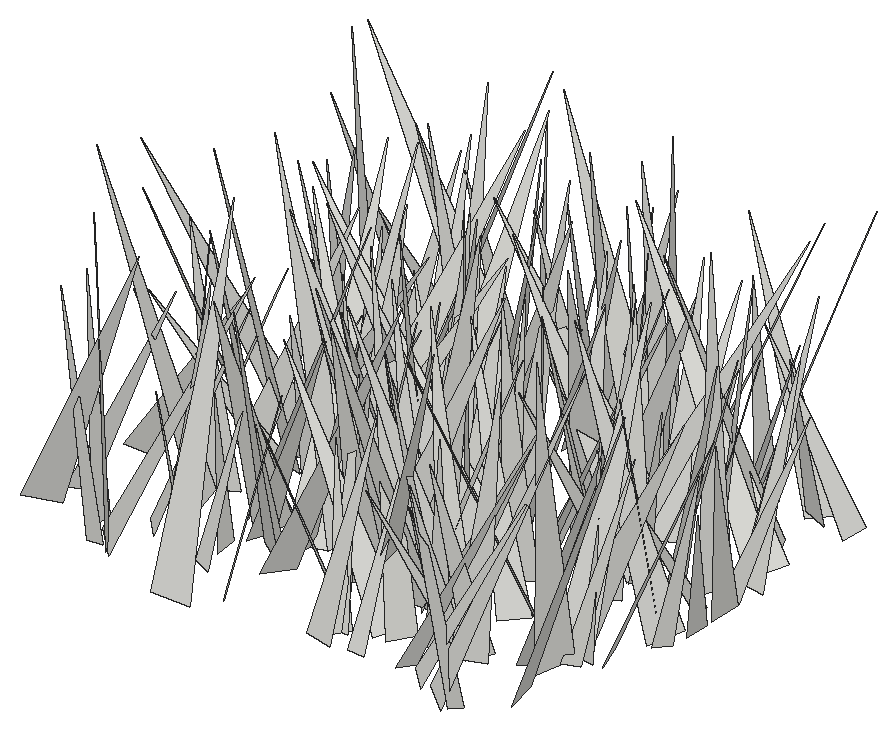
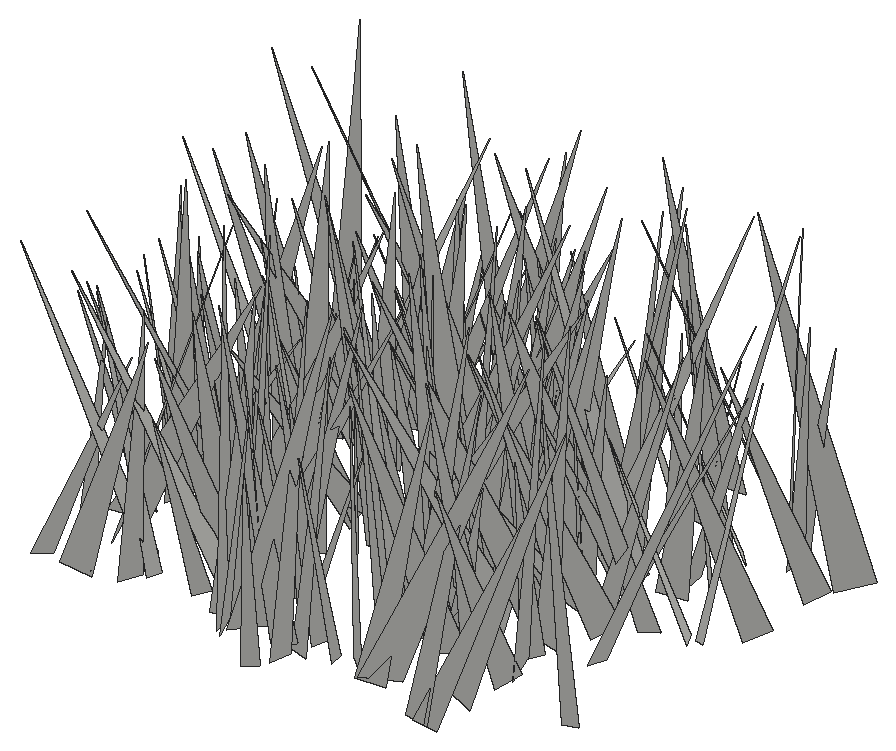
# SketchUp Ruby script. Lengths in inches.
U = 1.inch
M = Sketchup.active_model
def pt(a) = Geom::Point3d.new(a.map { |v| v * U })
def face(e, loops, mat)
  f = e.add_face(loops[0].map { |a| pt(a) })
  loops[1..].each { |l| e.add_face(l.map { |a| pt(a) }).erase! }
  f.material = f.back_material = mat if mat
  f
end
# faces: each face lists its corners as indices into pts; further lists are holes
def faces(e, pts, list, mat = nil) = list.each { |f| face(e, (f[0].is_a?(Array) ? f : [f]).map { |l| l.map { |i| pts[i] } }, mat) }
# xy, xz, yz: faces in a plane at the given z, y or x. An outline is a flat list of corners, or four numbers for a rectangle; further outlines are holes
def ring(l) = l.size == 4 ? [[l[0], l[1]], [l[2], l[1]], [l[2], l[3]], [l[0], l[3]]] : l.each_slice(2).to_a
def flat(e, list, mat, &to3) = list.each { |f| face(e, (f[0].is_a?(Array) ? f : [f]).map { |l| ring(l).map { |u, v| to3.(u, v) } }, mat) }
def xy(e, z, list, mat = nil) = flat(e, list, mat) { |x, y| [x, y, z] }
def xz(e, y, list, mat = nil) = flat(e, list, mat) { |x, z| [x, y, z] }
def yz(e, x, list, mat = nil) = flat(e, list, mat) { |y, z| [x, y, z] }
def lines(e, pts, list) = list.each { |a, b| e.add_line(pt(pts[a]), pt(pts[b])) }
# prism: a flat outline (further loops are holes) pulled along v
def prism(e, loops, v, mat = nil)
  f = face(e, loops, mat); d = Geom::Vector3d.new(v.map { |x| x * U })
  f.pushpull(f.normal.samedirection?(d) ? d.length : -d.length)
end
def box(e, o, s, mat = nil) = prism(e, [[o, [o[0] + s[0], o[1], o[2]], [o[0] + s[0], o[1] + s[1], o[2]], [o[0], o[1] + s[1], o[2]]]], [0, 0, s[2]], mat)
def at(x, y, z, deg = 0) = Geom::Transformation.translation(pt([x, y, z])) * Geom::Transformation.rotation(ORIGIN, Z_AXIS, deg.degrees)
def axes(o, x, y, z) = Geom::Transformation.new([*x, 0, *y, 0, *z, 0, *pt(o).to_a, 1])
def part(name) = M.definitions.add(name)
# library, detail: a bought-in or finely detailed component or shape, given as its bounding box
def library(name, o, s) = part(name).tap { |d| box(d.entities, o, s) }
def detail(e, o, s) = box(e.add_group.entities, o, s)
def put(e, d, t, mat = nil) = e.add_instance(d, t).tap { |i| i.material = mat if mat }
def group(e, t, mat = nil) = e.add_group.tap { |g| g.transformation = t; g.material = mat if mat }.entities
root = M.entities
c1 = part("fur_instance\#9")
p = [[0.8125,0,1.79],[0.67,-0.02,1.48],[0,-0.11,0],[0,0.11,0]]
faces(c1.entities,p,[[0,1,2,3]])
put(root,c1,axes([148.23,232.82,-27.1],[0.29151,4.89673,1.62599],[5.06271,0.04273,-1.03633],[0.99541,-1.65136,4.79468]))
put(root,c1,axes([153.89,233.59,-27.1],[-3.07283,-1.79032,0.75021],[-1.87261,3.10397,-0.26279],[0.51124,0.60869,3.54662]))
put(root,c1,axes([153.01,232.85,-27.1],[3.55975,3.91646,0.08522],[3.79537,-3.41954,-1.38552],[0.97011,-0.99289,5.10792]))
put(root,c1,axes([141.76,233.23,-27.1],[-3.37291,-1.64413,0.77782],[-1.79286,3.28135,-0.83849],[0.30629,1.10194,3.65741]))
put(root,c1,axes([141.93,231.76,-27.1],[-0.24232,8.0833,1.63068],[8.24361,0.27788,-0.15248],[0.20433,-1.625,8.08549]))
put(root,c1,axes([137.36,233.72,-27.1],[-5.46878,-3.64969,2.6695],[-4.02035,5.84198,-0.2491],[2.0696,1.70441,6.57007]))
put(root,c1,axes([154.51,232.05,-27.1],[4.64022,6.0526,0.40907],[6.0581,-4.59639,-0.71102],[0.31728,-0.75645,7.59342]))
put(root,c1,axes([133.34,234.75,-27.1],[5.01421,-5.55154,0.43768],[-5.45899,-4.78379,1.86233],[1.10028,1.565,7.24525]))
put(root,c1,axes([137.01,233.36,-27.1],[-2.00481,-4.221,2.16779],[-4.72189,1.54205,-1.3643],[-0.46899,2.51807,4.46932]))
put(root,c1,axes([155.55,231.93,-27.1],[-6.80362,-1.51626,0.05987],[-1.39466,6.13985,-2.9915],[-0.59797,2.93174,6.29597]))
put(root,c1,axes([148.56,233.77,-27.1],[-3.29969,1.99263,1.18367],[2.06312,3.46364,-0.07948],[1.05601,-0.54058,3.85386]))
put(root,c1,axes([152.93,235.59,-27.1],[-3.89152,-1.38284,0.09587],[-1.31779,3.77936,1.02238],[0.42995,-0.93252,4.00136]))
put(root,c1,axes([153.84,235.57,-27.1],[3.33283,-3.55166,1.19436],[-3.37517,-3.53973,-1.10774],[-1.62758,0.06765,4.74288]))
put(root,c1,axes([143.4,233.2,-27.1],[3.40494,2.47984,0.75094],[2.39973,-3.48584,0.63038],[-0.97714,0.08048,4.16483]))
put(root,c1,axes([152.64,235.5,-27.1],[-3.58815,0.95471,1.93369],[1.59157,3.70529,1.12394],[1.45517,-1.69849,3.5388]))
put(root,c1,axes([148.56,235.94,-27.1],[7.85727,-0.11013,0.63762],[0.0287,-7.70188,-1.68396],[-0.64642,-1.6806,7.67549]))
put(root,c1,axes([156.96,234.15,-27.1],[7.02887,1.41814,0.69885],[1.44367,-7.05544,-0.2028],[-0.64447,-0.3379,7.16763]))
put(root,c1,axes([149.99,232.86,-27.1],[0.7,4.04155,0.09862],[4.02713,-0.70587,0.34334],[-0.35517,-0.03822,4.08733]))
put(root,c1,axes([137.3,233.7,-27.1],[4.92095,5.18553,0.33695],[5.09859,-4.72846,-1.69263],[1.00379,-1.4039,6.94554]))
put(root,c1,axes([152.1,233.29,-27.1],[5.39304,-0.33096,0.39775],[-0.43435,-5.15892,1.59671],[-0.28121,1.6213,5.16187]))
put(root,c1,axes([148,234.76,-27.1],[-3.22375,-2.36609,0.00506],[-2.25529,3.0702,-1.21594],[-0.71558,0.9831,3.80952]))
put(root,c1,axes([152.02,235.3125,-27.1],[3.93082,-2.70083,1.38603],[-2.7651,-4.12134,-0.18897],[-1.2529,0.6221,4.76552]))
put(root,c1,axes([139.46,235.18,-27.1],[-0.7765,-5.95979,2.50914],[-6.25232,1.3369,1.24057],[1.65027,2.26084,5.88073]))
put(root,c1,axes([136.2,234.75,-27.1],[-5.05567,-0.39861,1.84756],[-0.46846,5.37567,-0.1221],[1.83109,0.27472,5.06989]))
put(root,c1,axes([148.35,233.79,-27.1],[0.28645,5.00767,1.03913],[5.08565,-0.389,0.47271],[-0.54104,-1.00525,4.99354]))
put(root,c1,axes([141.27,234.49,-27.1],[1.148,3.43718,0.90942],[3.54891,-1.0498,-0.51218],[0.21566,-1.0212,3.58745]))
put(root,c1,axes([149.99,234.9375,-27.1],[-4.53112,4.00144,0.54603],[3.94801,4.21612,1.86503],[-0.85024,-1.74745,5.75015]))
put(root,c1,axes([153.67,235.1,-27.1],[3.4619,-5.09824,2.22403],[-5.52391,-3.4582,0.67108],[-0.65172,2.22978,6.12588]))
put(root,c1,axes([156.52,236.71,-27.1],[6.94101,-3.43299,1.84422],[-3.2352,-7.17632,-1.18245],[-2.17258,-0.28153,7.65277]))
put(root,c1,axes([142.72,236.91,-27.1],[-2.91514,-5.53327,1.42514],[-5.42873,3.18122,1.24695],[1.78243,0.63944,6.12864]))
put(root,c1,axes([141.09,236.17,-27.1],[3.87563,-0.57439,1.14349],[-0.32332,-3.96837,-0.89752],[-1.23813,-0.76168,3.81378]))
put(root,c1,axes([147.22,237.29,-27.1],[1.68994,-6.65431,0.98946],[-6.7239,-1.70391,0.02495],[-0.21912,0.96522,6.8655]))
put(root,c1,axes([149.86,237.21,-27.1],[-1.24664,-7.42641,1.30497],[-7.49381,1.07378,-1.04811],[-0.83512,1.45053,7.45702]))
put(root,c1,axes([141.66,238.41,-27.1],[5.49992,-4.64771,0.52674],[-4.40214,-5.41809,-1.84207],[-1.58109,-1.08206,6.96111]))
put(root,c1,axes([152.46,236.4,-27.1],[-7.15146,0.58689,0.88826],[0.71619,7.11549,1.06478],[0.78773,-1.14116,7.09606]))
put(root,c1,axes([155.46,237.81,-27.1],[-4.1792,-5.61615,0.15739],[-5.61189,4.16336,-0.45249],[-0.26934,0.3962,6.98585]))
put(root,c1,axes([143.77,235.97,-27.1],[7.07032,-2.50038,0.22823],[-2.5064,-6.98854,1.08245],[0.14815,1.09629,7.42089]))
put(root,c1,axes([143.08,236.97,-27.1],[-3.69542,-5.95234,1.80806],[-6.20183,3.68953,-0.52934],[0.48649,1.82006,6.98615]))
put(root,c1,axes([146.64,236.37,-27.1],[-2.09497,-3.98677,2.51489],[-4.46346,2.56262,0.34425],[1.51546,2.03632,4.49052]))
put(root,c1,axes([137.96,235.66,-27.1],[3.6626,3.70148,0.35684],[3.71844,-3.64024,-0.40601],[0.03906,-0.53912,5.19141]))
put(root,c1,axes([150.67,234.82,-27.1],[-7.44461,1.33123,0.56849],[1.18187,7.30967,-1.63995],[0.83578,1.52121,7.38274]))
put(root,c1,axes([141.6,237.66,-27.1],[5.62437,-1.82953,0.08499],[-1.8284,-5.62476,-0.0835],[-0.10665,-0.05312,5.91386]))
put(root,c1,axes([133.94,236.26,-27.1],[4.38543,-2.43855,0.87514],[-2.59033,-4.09309,1.5752],[0.05089,1.80126,4.76417]))
put(root,c1,axes([142.1,239.125,-27.1],[-4.63636,-6.55031,0.51962],[-6.56307,4.58532,-0.75728],[-0.32055,0.86066,7.9893]))
put(root,c1,axes([138.32,238.4375,-27.1],[-7.66466,-1.90179,1.421],[-1.79066,7.78455,0.75987],[1.55871,-0.40873,7.86043]))
put(root,c1,axes([147.3125,238.78,-27.1],[-0.33805,-5.61743,0.95415],[-5.65981,0.22074,-0.70569],[-0.6576,0.9879,5.58317]))
put(root,c1,axes([146.99,238.02,-27.1],[-2.52237,2.99386,0.77548],[2.99232,2.10973,1.58806],[-0.78138,-1.58517,3.57821]))
put(root,c1,axes([151.04,237.625,-27.1],[3.04965,-4.5466,3.26672],[-5.09549,-3.79519,-0.52522],[-2.31926,2.35973,5.44941]))
put(root,c1,axes([150.29,237.89,-27.1],[4.26333,-3.02404,0.31767],[-2.97687,-4.03955,1.49732],[0.61963,1.39963,5.00788]))
put(root,c1,axes([137.4,238.39,-27.1],[4.80931,3.10321,2.02961],[3.46778,-4.94111,-0.66234],[-1.31293,-1.68352,5.68513]))
put(root,c1,axes([147.29,239.39,-27.1],[-7.26006,2.55391,1.83228],[2.95803,7.11093,1.80912],[1.0629,-2.34529,7.48051]))
put(root,c1,axes([149.7,239.41,-27.1],[-4.06839,-1.50308,0.30492],[-1.46625,4.06536,0.47647],[0.44983,-0.34301,4.31092]))
put(root,c1,axes([149.56,237.4,-27.1],[4.3993,3.63087,0.47155],[3.65139,-4.40515,-0.14642],[-0.27004,-0.41338,5.70225]))
put(root,c1,axes([143.54,237.99,-27.1],[4.7353,0.6555,1.15241],[0.55235,-4.8611,0.49538],[-1.20525,0.34759,4.75472]))
put(root,c1,axes([157.65,238.6,-27.1],[5.84375,1.80801,0.13219],[1.81029,-5.79638,-0.74876],[0.09603,-0.75425,6.07105]))
put(root,c1,axes([140.02,239.42,-27.1],[8.09633,1.85359,0.38508],[1.89305,-7.94545,-1.5559],[-0.02113,-1.6027,8.15877]))
put(root,c1,axes([146.75,238.73,-27.1],[1.17731,-6.81979,2.88625],[-6.91612,0.0321,2.89694],[2.64712,3.11697,6.28517]))
put(root,c1,axes([156.87,237.23,-27.1],[3.7026,-0.58317,1.91769],[-1.4169,-3.61072,1.63767],[-1.41775,2.08554,3.37155]))
put(root,c1,axes([144.97,239.95,-27.1],[-5.38028,-3.08502,1.66928],[-3.07413,5.61908,0.47644],[1.68926,0.39986,6.18367]))
put(root,c1,axes([157.23,237.8,-27.1],[1.77865,4.09096,1.0407],[3.89915,-2.02489,1.29578],[-1.61729,-0.38272,4.26855]))
put(root,c1,axes([146.23,237.67,-27.1],[3.62964,3.56201,0.97293],[3.43547,-3.75775,0.94107],[-1.35352,0.01415,4.99765]))
put(root,c1,axes([138.33,239.55,-27.1],[1.39978,-5.30319,2.32473],[-5.64349,-1.78474,-0.67328],[-1.29585,2.04412,5.44334]))
put(root,c1,axes([153.04,238.625,-27.1],[-3.19469,4.99874,1.10839],[5.10889,3.02549,1.08057],[-0.33936,-1.5103,5.83317]))
put(root,c1,axes([155.4,239.77,-27.1],[1.83372,-5.8574,1.52699],[-5.60076,-1.03656,2.74963],[2.29617,2.14936,5.48737]))
put(root,c1,axes([135.29,241.7,-27.1],[-2.98193,-4.15353,0.46379],[-3.81224,2.9367,1.78925],[1.71281,-0.69483,4.78981]))
put(root,c1,axes([144.36,242.33,-27.1],[-0.43827,-6.52973,0.002],[-6.42899,0.43186,1.145],[1.14256,-0.07472,6.44348]))
put(root,c1,axes([133.84,239.99,-27.1],[3.57334,-4.4658,0.19156],[-4.12422,-3.19939,2.34597],[1.72363,1.60293,5.21618]))
put(root,c1,axes([146.41,238.24,-27.1],[-6.04879,4.39479,0.23194],[4.40071,6.03643,0.38865],[-0.04117,-0.45072,7.46666]))
put(root,c1,axes([144.76,241.12,-27.1],[1.52104,-3.59534,0.18519],[-3.58042,-1.53172,-0.32978],[-0.37596,0.04131,3.88989]))
put(root,c1,axes([144.45,239.28,-27.1],[-8.05212,1.79962,1.36323],[1.82873,8.16018,0.02927],[1.32393,-0.32629,8.25072]))
put(root,c1,axes([156.2,238.23,-27.1],[-1.91497,6.86191,1.78883],[6.91485,2.21764,-1.10438],[1.57179,-1.39609,7.03799]))
put(root,c1,axes([146.48,237.67,-27.1],[-5.7713,0.32455,0.04644],[0.28097,5.31808,-2.2482],[0.16895,2.24233,5.3253]))
put(root,c1,axes([155.48,236.08,-27.1],[6.83312,3.40706,1.30672],[2.45514,-6.34476,3.70451],[-2.69961,2.8536,6.67654]))
put(root,c1,axes([138.86,242.26,-27.1],[-4.92347,-1.39259,0.14711],[-1.23579,4.5738,1.93769],[0.65861,-1.82825,4.73553]))
put(root,c1,axes([147.97,239.34,-27.1],[-5.43325,1.77797,0.85582],[1.73658,5.49897,-0.39929],[0.93695,0.1182,5.7028]))
put(root,c1,axes([158.37,241.09,-27.1],[-6.07802,2.92755,1.98205],[3.37511,5.97833,1.51972],[1.05246,-2.26504,6.57292]))
put(root,c1,axes([151.33,241.09,-27.1],[-3.30956,4.62511,3.28339],[5.43338,3.67626,0.29816],[1.62808,-2.86687,5.67942]))
put(root,c1,axes([146.87,241.35,-27.1],[-1.94061,6.26278,4.61542],[7.19839,3.24975,-1.38302],[2.95087,-3.80883,6.40903]))
put(root,c1,axes([144.56,240.59,-27.1],[0.81184,5.62301,2.88886],[5.96448,-1.64652,1.52868],[-2.09495,-2.50871,5.47179]))
put(root,c1,axes([158.71,240.47,-27.1],[3.49135,-1.63355,1.08284],[-1.80913,-3.53699,0.49727],[-0.7537,0.9229,3.8224]))
put(root,c1,axes([159,242.1875,-27.1],[3.9114,-1.46291,0.01114],[-1.40736,-3.77134,-1.11157],[-0.39945,-1.03737,4.02536]))
put(root,c1,axes([140.84,241.93,-27.1],[2.96444,-3.24193,0.90441],[-3.19075,-3.09049,-0.61962],[-1.07107,0.23387,4.34903]))
put(root,c1,axes([148.3125,242.3,-27.1],[-7.32197,2.2534,1.35544],[2.57225,6.97064,2.30649],[0.54639,-2.61889,7.30542]))
put(root,c1,axes([154.31,243.56,-27.1],[-5.03232,-2.4099,0.87584],[-1.92345,4.82363,2.22078],[1.6956,-1.68045,5.11859]))
put(root,c1,axes([156.44,242.84,-27.1],[-3.5454,-4.09399,1.47684],[-3.82101,3.83994,1.47185],[2.08366,0.07566,5.21193]))
put(root,c1,axes([145.8125,242.33,-27.1],[3.71105,4.69804,3.51461],[5.68502,-3.90755,-0.77947],[-1.45074,-3.29476,5.93598]))
put(root,c1,axes([139.26,240.61,-27.1],[4.45979,0.0367,0.09292],[0.01604,-4.35825,0.95137],[-0.0986,0.95079,4.35729]))
put(root,c1,axes([141.31,241.28,-27.1],[2.46567,3.17158,1.58955],[3.37143,-2.69731,0.15219],[-1.10413,-1.15357,4.01439]))
put(root,c1,axes([154.62,241.98,-27.1],[3.53738,-5.32848,1.99163],[-5.66565,-3.51029,0.67133],[-0.50966,2.039,6.36044]))
put(root,c1,axes([150.43,241.44,-27.1],[6.68807,0.43229,0.66728],[0.41432,-6.71942,0.20043],[-0.67859,0.15798,6.69903]))
put(root,c1,axes([143.47,238.09,-27.1],[-6.01479,5.28528,0.0687],[5.03484,5.76049,-2.36301],[1.60915,1.73181,7.65037]))
put(root,c1,axes([143.72,244.72,-27.1],[5.51839,-2.97407,0.09463],[-2.75984,-5.19025,-2.17974],[-1.11235,-1.87694,5.87762]))
put(root,c1,axes([143.98,241.42,-27.1],[0.77097,6.55392,2.92574],[6.60675,-1.79779,2.28627],[-2.8044,-2.43357,6.19042]))
put(root,c1,axes([158.96,243.92,-27.1],[5.13341,-1.95182,0.40555],[-1.78394,-4.9977,-1.47188],[-0.88973,-1.24068,5.29103]))
put(root,c1,axes([146.28,241.48,-27.1],[4.52049,-0.19473,1.20973],[-0.39564,-4.60837,0.73662],[-1.15967,0.81315,4.46432]))
put(root,c1,axes([145.81,240.43,-27.1],[-1.08496,4.24211,0.2137],[4.12597,1.10497,-0.98676],[1.00871,0.04308,4.26602]))
put(root,c1,axes([135.72,241.8,-27.1],[3.83341,2.26597,0.28943],[2.28132,-3.82668,-0.25597],[-0.11822,-0.36786,4.44568]))
put(root,c1,axes([139.32,242.45,-27.1],[-3.64938,-5.29226,1.74557],[-5.55344,3.28039,-1.66476],[-0.463,2.36729,6.20923]))
put(root,c1,axes([144.82,242.91,-27.1],[5.44749,2.02001,0.26599],[2.02291,-5.27178,-1.39377],[0.24298,-1.39796,5.64031]))
put(root,c1,axes([150.3,241.73,-27.1],[0.9151,5.15761,1.58711],[5.35443,-1.06795,0.38322],[-0.67079,-1.48856,5.22413]))
put(root,c1,axes([152.88,243.61,-27.1],[3.69815,0.46024,1.83595],[1.02421,-3.87534,-1.09159],[-1.5917,-1.42435,3.56322]))
put(root,c1,axes([137.25,242.25,-27.1],[1.94999,6.06367,1.85826],[6.06829,-1.21894,-2.39034],[1.84311,-2.40204,5.90397]))
put(root,c1,axes([137.34,245.29,-27.1],[-7.29024,-1.74958,0.87658],[-1.40156,7.02793,2.37084],[1.36568,-2.12702,7.11251]))
put(root,c1,axes([142.7,242.08,-27.1],[-2.8521,5.31504,2.52319],[5.50682,3.39878,-0.93481],[2.07151,-1.71732,5.95905]))
put(root,c1,axes([158,243.6,-27.1],[-0.53868,-3.7535,0.51973],[-3.36849,0.23389,-1.80211],[-1.73555,0.71104,3.33637]))
put(root,c1,axes([151.36,242.1875,-27.1],[3.9948,0.59542,0.26899],[0.55235,-3.96784,0.58004],[-0.34899,0.53573,3.99706]))
put(root,c1,axes([152.68,244.03,-27.1],[-4.88015,-2.78524,1.52655],[-2.68194,5.11285,0.7548],[1.7015,0.07051,5.5681]))
put(root,c1,axes([154.36,241.78,-27.1],[4.62309,3.63215,1.82021],[3.50208,-4.96051,1.00367],[-2.05939,-0.28182,5.79293]))
put(root,c1,axes([147.66,243.18,-27.1],[-6.42815,4.45601,0.04956],[4.21627,6.0534,2.59983],[-1.44275,-2.16333,7.37686]))
put(root,c1,axes([151.31,245.56,-27.1],[4.3126,-6.65441,0.44802],[-6.65528,-4.32849,-0.22777],[-0.435,0.25174,7.9264]))
put(root,c1,axes([147.5625,242.64,-27.1],[-5.47988,-2.79163,2.54101],[-3.31815,5.69792,-0.89593],[1.79996,2.00489,6.08438]))
put(root,c1,axes([154.83,243.97,-27.1],[4.24921,-1.39082,0.67887],[-1.35455,-4.30166,-0.33452],[-0.74864,-0.11098,4.4585]))
put(root,c1,axes([156.4375,244.01,-27.1],[5.73568,-0.06882,1.05766],[0.01363,-5.81521,-0.45231],[-1.05981,-0.44725,5.71823]))
put(root,c1,axes([138.55,243.24,-27.1],[4.87522,-3.55324,0.35007],[-3.38958,-4.41978,2.34354],[1.12198,2.08707,5.55888]))
put(root,c1,axes([154.69,244.45,-27.1],[-6.88709,2.46248,0.81316],[2.58785,6.67518,1.70354],[0.16756,-1.88022,7.11293]))
put(root,c1,axes([141.51,241.94,-27.1],[3.64416,1.65962,0.06909],[1.4569,-3.27351,1.789],[-0.79783,1.60274,3.58241]))
put(root,c1,axes([149.46,244.64,-27.1],[4.52719,2.71843,2.25301],[3.1828,-4.72799,-0.69084],[-1.52829,-1.79378,5.23527]))
put(root,c1,axes([156.55,243.59,-27.1],[4.95919,2.18923,1.00137],[2.21006,-5.04934,0.09393],[-0.95452,-0.31696,5.4201]))
put(root,c1,axes([149.01,243.7,-27.1],[1.36969,7.27883,2.41401],[7.66649,-1.2409,-0.6083],[0.18385,-2.48268,7.38156]))
put(root,c1,axes([143.18,244.73,-27.1],[4.24569,0.44069,0.96407],[0.53821,-4.32495,-0.39327],[-0.91322,-0.50013,4.25034]))
put(root,c1,axes([146.86,243.6,-27.1],[3.58302,-2.92408,2.58959],[-3.63927,-3.77537,0.77237],[-1.41842,2.30013,4.5598]))
put(root,c1,axes([139.69,245.42,-27.1],[1.75829,5.41715,3.42251],[6.36736,-1.87488,-0.30363],[-0.71818,-3.36006,5.68726]))
put(root,c1,axes([141.34,243.84,-27.1],[2.97178,5.39968,0.42783],[5.06638,-2.59832,-2.39825],[1.91609,-1.5044,5.67771]))
put(root,c1,axes([146.77,244.67,-27.1],[4.56446,-0.76979,0.5853],[-0.81155,-4.58493,0.29877],[-0.52586,0.39409,4.61927]))
put(root,c1,axes([146,245.93,-27.1],[4.04324,-6.81137,0.9787],[-6.74817,-3.70246,2.11055],[1.34718,1.89668,7.63467]))
put(root,c1,axes([151.41,242.125,-27.1],[5.35308,0.77922,1.1136],[0.09871,-4.73607,2.83947],[-1.35556,2.73224,4.60435]))
put(root,c1,axes([141.13,242.44,-27.1],[1.53253,6.73152,0.42824],[6.72346,-1.5597,0.45586],[-0.5402,-0.31526,6.8887]))
put(root,c1,axes([143.18,247.01,-27.1],[7.23074,-0.77372,0.74856],[-0.57311,-7.06946,-1.77111],[-0.91134,-1.69312,7.05304]))
put(root,c1,axes([157.55,245.0625,-27.1],[6.19428,-1.57461,3.33029],[-1.87234,-6.95675,0.19327],[-3.17247,1.03131,6.38836]))
put(root,c1,axes([158.33,245.17,-27.1],[1.81296,4.05322,0.9149],[4.0683,-1.5284,-1.29051],[0.84535,-1.3371,4.24853]))
put(root,c1,axes([156.49,245.0625,-27.1],[4.35259,2.65064,0.87547],[2.69973,-4.40951,-0.0717],[-0.70982,-0.51745,5.09567]))
put(root,c1,axes([151.92,246.72,-27.1],[-3.79405,-1.81524,0.00607],[-1.81515,3.79397,0.03081],[0.01877,-0.02517,4.20582]))
put(root,c1,axes([153.38,245.53,-27.1],[-1.15441,5.11883,1.74969],[5.40957,1.09949,0.35248],[0.0216,-1.78472,5.23554]))
put(root,c1,axes([141.09,244.12,-27.1],[-0.22471,7.89617,1.63504],[7.5306,0.79034,-2.78188],[2.88322,-1.44886,7.39332]))
put(root,c1,axes([143.38,246.6,-27.1],[1.79677,-5.19077,1.98742],[-5.55817,-1.66844,0.66734],[0.02536,2.09632,5.45226]))
put(root,c1,axes([144.99,244.83,-27.1],[-0.16365,8.04006,1.71484],[8.20749,0.06185,0.49328],[-0.46944,-1.72152,8.02659]))
put(root,c1,axes([151.82,245.68,-27.1],[1.21689,3.56799,0.58582],[3.55761,-1.29191,0.47847],[-0.64586,-0.39367,3.73931]))
put(root,c1,axes([143.25,246.25,-27.1],[-2.90723,2.3787,0.42473],[2.40963,2.90345,0.23285],[0.1797,-0.4498,3.74913]))
put(root,c1,axes([158.53,246.05,-27.1],[0.17579,4.7582,1.26729],[4.89735,-0.03702,-0.54033],[0.51227,-1.27889,4.73069]))
put(root,c1,axes([139.47,246.51,-27.1],[-3.40994,2.09099,1.78678],[2.1335,3.80705,-0.3836],[1.73581,-0.57158,3.98156]))
put(root,c1,axes([152.39,247.19,-27.1],[-4.17203,-5.0841,2.64194],[-5.48144,4.49304,-0.00972],[1.66784,2.04897,6.57676]))
put(root,c1,axes([143.81,248.875,-27.1],[7.53646,1.85279,1.2332],[2.16443,-7.11553,-2.53698],[-0.51849,-2.77277,7.33449]))
put(root,c1,axes([156.35,246.67,-27.1],[3.88828,4.27161,1.82836],[4.44707,-4.1121,0.14976],[-1.3465,-1.2459,5.77433]))
put(root,c1,axes([151.5,248.45,-27.1],[-6.98354,0.71492,0.27676],[0.75932,6.7998,1.59491],[0.10557,-1.6153,6.83646]))
put(root,c1,axes([157.6,248.95,-27.1],[-6.20771,-3.16783,0.82777],[-3.08728,6.25411,0.78157],[1.09042,-0.32718,6.92531]))
put(root,c1,axes([149.4,248.6875,-27.1],[-6.05597,0.77226,2.0179],[1.21073,6.18666,1.26588],[1.78953,-1.57224,5.97233]))
put(root,c1,axes([152.47,246.11,-27.1],[3.82071,6.83533,0.31448],[6.59967,-3.58608,-2.23672],[1.80694,-1.35528,7.50444]))
put(root,c1,axes([143.7,248.06,-27.1],[-6.59669,1.20746,2.1658],[1.44471,6.87425,0.5679],[2.0153,-0.97558,6.6822]))
put(root,c1,axes([142.8,245.91,-27.1],[-0.26987,6.47949,0.83868],[6.52839,0.23411,0.29205],[-0.25936,-0.84936,6.47853]))
put(root,c1,axes([139.26,247.49,-27.1],[-7.32615,-2.19993,2.60741],[-2.57876,7.61493,-0.82074],[2.23345,1.57604,7.60517]))
put(root,c1,axes([158.22,247.4375,-27.1],[-5.28258,5.45364,0.12335],[5.18528,4.96674,2.47132],[-1.69419,-1.80343,7.17917]))
put(root,c1,axes([153.84,246.93,-27.1],[3.74309,-3.05687,3.19875],[-4.02453,-4.09315,0.7978],[-1.83838,2.73658,4.76642]))
put(root,c1,axes([158.2,246.35,-27.1],[1.54833,5.59255,0.52827],[5.59137,-1.58705,0.41342],[-0.54067,-0.39706,5.78818]))
put(root,c1,axes([150.07,249.32,-27.1],[2.36521,-5.47601,0.71506],[-5.30162,-2.03369,1.96193],[1.54624,1.40343,5.6331]))
put(root,c1,axes([135.09,249.74,-27.1],[-1.49518,-5.85947,1.8909],[-5.5495,2.12534,2.19783],[2.66683,1.13753,5.63369]))
put(root,c1,axes([141.99,244.88,-27.1],[7.42778,3.7642,0.92799],[3.25227,-7.14156,2.93652],[-2.11023,2.24305,7.79217]))
put(root,c1,axes([148.11,249.21,-27.1],[-3.79704,-0.30553,0.54536],[-0.26679,3.82814,0.28712],[0.56533,-0.2455,3.79848]))
put(root,c1,axes([141.41,247.65,-27.1],[-2.96108,3.10315,0.36366],[3.04624,2.97875,-0.6142],[0.69442,0.16515,4.24503]))
put(root,c1,axes([148.73,248.33,-27.1],[-3.00951,3.51493,1.30262],[3.55292,3.20728,-0.44587],[1.1951,-0.68362,4.60577]))
put(root,c1,axes([153.36,247.44,-27.1],[-2.46279,4.53865,0.90199],[4.34757,2.61941,-1.3098],[1.58479,-0.13272,4.99491]))
put(root,c1,axes([154.54,250.47,-27.1],[5.4983,0.81734,0.21266],[0.84397,-5.26527,-1.58403],[0.03145,-1.59793,5.32824]))
put(root,c1,axes([144.1,249.74,-27.1],[5.56182,2.46032,2.03104],[2.73268,-5.78042,-0.48104],[-1.64644,-1.28288,6.06264]))
put(root,c1,axes([139.67,250.79,-27.1],[-1.62801,-6.13851,1.48062],[-6.15059,1.19536,-1.80699],[-1.42958,1.84764,6.08822]))
put(root,c1,axes([146.36,250.52,-27.1],[5.46664,-0.56538,0.68203],[-0.51758,-5.49848,-0.40957],[-0.71898,-0.34055,5.48051]))
put(root,c1,axes([157.04,251.74,-27.1],[-0.66532,-4.77379,0.4836],[-4.67341,0.75535,1.0268],[1.0873,0.32553,4.70929]))
put(root,c1,axes([153.01,248.41,-27.1],[6.48449,2.8801,0.19854],[2.8437,-6.45643,0.78158],[-0.49773,0.63448,7.05214]))
put(root,c1,axes([142.17,248.2,-27.1],[-2.25135,6.36064,1.32657],[6.19225,2.52565,-1.60099],[1.96812,-0.67041,6.55463]))
put(root,c1,axes([138.99,248.59,-27.1],[-4.17558,2.72173,1.55923],[2.19552,4.39009,-1.78362],[2.24025,0.77057,4.65424]))
put(root,c1,axes([146.53,251.78,-27.1],[-2.50316,-5.2047,1.47138],[-5.2002,2.76171,0.92225],[1.48721,0.89649,5.70124]))
put(root,c1,axes([143.03,251.83,-27.1],[1.51569,-5.39227,1.25729],[-5.41404,-1.71643,-0.83467],[-1.15995,0.96539,5.5387]))
put(root,c1,axes([155.1,251.23,-27.1],[-4.81176,0.83188,2.6308],[1.27412,5.3609,0.63523],[2.44739,-1.15538,4.84165]))
put(root,c1,axes([152.3,250.42,-27.1],[2.6099,-2.39325,0.8726],[-2.54736,-2.4537,0.88934],[-0.00348,1.24593,3.42758]))
put(root,c1,axes([150.16,251.68,-27.1],[7.38345,1.68053,2.79244],[2.22073,-7.65548,-1.26461],[-2.38543,-1.92527,7.46594]))
put(root,c1,axes([149.39,250,-27.1],[-4.16278,-2.64249,2.71758],[-3.23685,4.57857,-0.50613],[1.97251,1.93665,4.90462]))
put(root,c1,axes([150.39,251.27,-27.1],[1.19646,-6.35488,2.45253],[-6.76034,-1.41301,-0.36331],[-0.83491,2.33448,6.45631]))
put(root,c1,axes([142.91,251.41,-27.1],[-7.09229,4.18803,1.11711],[4.32642,6.70959,2.31334],[-0.26383,-2.55536,7.90497]))
put(root,c1,axes([158.95,251.74,-27.1],[-4.51725,1.3418,0.80765],[1.52463,4.33149,1.33117],[0.35811,-1.51528,4.52039]))
put(root,c1,axes([146.88,252.46,-27.1],[6.67439,0.3641,2.55328],[0.99441,-6.8993,-1.61558],[-2.3797,-1.86182,6.48614]))
put(root,c1,axes([147.42,251.54,-27.1],[0.1838,-6.38239,2.38865],[-6.46729,0.58989,2.0738],[2.14821,2.32195,6.03888]))
put(root,c1,axes([139.86,253.04,-27.1],[-1.86711,-6.21996,0.83765],[-6.21183,1.95621,0.67975],[0.89595,0.60083,6.45848]))
put(root,c1,axes([145.15,251.28,-27.1],[3.94564,1.0984,0.79467],[1.2,-3.96752,-0.47419],[-0.63087,-0.67703,4.06813]))
put(root,c1,axes([155.21,249.79,-27.1],[6.72288,3.05704,0.61475],[3.02645,-6.7488,0.46346],[-0.75102,0.16938,7.37074]))
put(root,c1,axes([149.29,251.44,-27.1],[-7.00283,2.97011,1.6591],[3.21934,7.01289,1.03394],[1.10002,-1.61605,7.53606]))
put(root,c1,axes([139.37,253.15,-27.1],[1.40326,-4.201,0.43994],[-3.89786,-1.46649,-1.57071],[-1.62745,-0.10993,4.1413]))
put(root,c1,axes([144.1875,251.19,-27.1],[3.38997,4.6985,2.258],[4.82742,-3.84601,0.75539],[-1.96736,-1.34115,5.74432]))
put(root,c1,axes([150,251.9,-27.1],[-4.89428,-1.48699,1.50253],[-1.73277,4.99254,-0.70337],[1.21087,1.13406,5.0666]))
put(root,c1,axes([157.14,251.96,-27.1],[-2.40654,5.51072,1.54274],[5.60544,1.9331,1.83892],[-1.15197,-2.10585,5.72519]))
put(root,c1,axes([147.37,253.66,-27.1],[0.94706,-3.59902,0.23008],[-3.53322,-0.8783,0.80484],[0.72266,0.42244,3.63347]))
